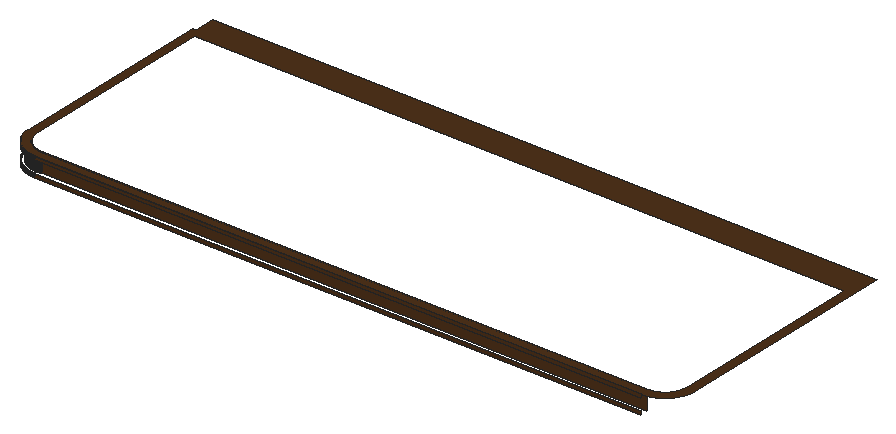
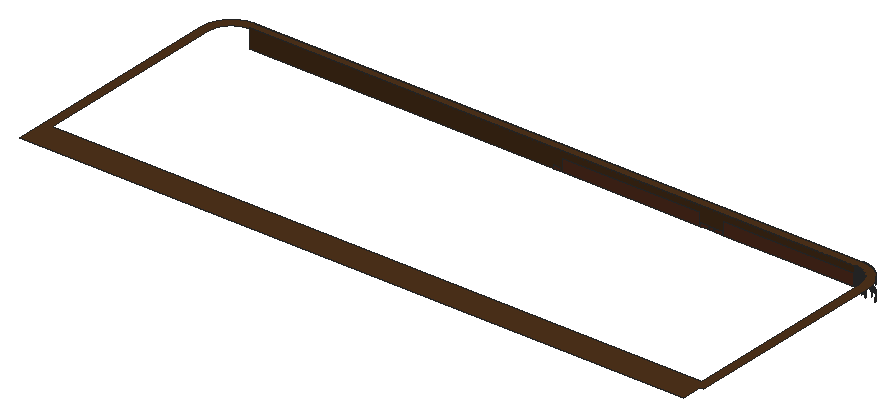
# SketchUp Ruby script. Lengths in inches.
U = 1.inch
M = Sketchup.active_model
def pt(a) = Geom::Point3d.new(a.map { |v| v * U })
def face(e, loops, mat)
  f = e.add_face(loops[0].map { |a| pt(a) })
  loops[1..].each { |l| e.add_face(l.map { |a| pt(a) }).erase! }
  f.material = f.back_material = mat if mat
  f
end
# faces: each face lists its corners as indices into pts; further lists are holes
def faces(e, pts, list, mat = nil) = list.each { |f| face(e, (f[0].is_a?(Array) ? f : [f]).map { |l| l.map { |i| pts[i] } }, mat) }
# xy, xz, yz: faces in a plane at the given z, y or x. An outline is a flat list of corners, or four numbers for a rectangle; further outlines are holes
def ring(l) = l.size == 4 ? [[l[0], l[1]], [l[2], l[1]], [l[2], l[3]], [l[0], l[3]]] : l.each_slice(2).to_a
def flat(e, list, mat, &to3) = list.each { |f| face(e, (f[0].is_a?(Array) ? f : [f]).map { |l| ring(l).map { |u, v| to3.(u, v) } }, mat) }
def xy(e, z, list, mat = nil) = flat(e, list, mat) { |x, y| [x, y, z] }
def xz(e, y, list, mat = nil) = flat(e, list, mat) { |x, z| [x, y, z] }
def yz(e, x, list, mat = nil) = flat(e, list, mat) { |y, z| [x, y, z] }
def lines(e, pts, list) = list.each { |a, b| e.add_line(pt(pts[a]), pt(pts[b])) }
# prism: a flat outline (further loops are holes) pulled along v
def prism(e, loops, v, mat = nil)
  f = face(e, loops, mat); d = Geom::Vector3d.new(v.map { |x| x * U })
  f.pushpull(f.normal.samedirection?(d) ? d.length : -d.length)
end
def box(e, o, s, mat = nil) = prism(e, [[o, [o[0] + s[0], o[1], o[2]], [o[0] + s[0], o[1] + s[1], o[2]], [o[0], o[1] + s[1], o[2]]]], [0, 0, s[2]], mat)
def at(x, y, z, deg = 0) = Geom::Transformation.translation(pt([x, y, z])) * Geom::Transformation.rotation(ORIGIN, Z_AXIS, deg.degrees)
def axes(o, x, y, z) = Geom::Transformation.new([*x, 0, *y, 0, *z, 0, *pt(o).to_a, 1])
def part(name) = M.definitions.add(name)
# library, detail: a bought-in or finely detailed component or shape, given as its bounding box
def library(name, o, s) = part(name).tap { |d| box(d.entities, o, s) }
def detail(e, o, s) = box(e.add_group.entities, o, s)
def put(e, d, t, mat = nil) = e.add_instance(d, t).tap { |i| i.material = mat if mat }
def group(e, t, mat = nil) = e.add_group.tap { |g| g.transformation = t; g.material = mat if mat }.entities
root = M.entities
M.materials.add("1799 AP 8574 BURNISHED CARAMEL").color = [140, 96, 69]
M.materials.add("1816 AP K197 Dark Kaapi-N").color = [79, 50, 27]
M.materials.add("[Wood Cherry Original]1").color = [93, 50, 33]
xy(root,401,[[[65.76,78,420.24,78,420.47,78.01,420.71,78.01,420.94,78.02,421.18,78.04,421.41,78.06,421.65,78.08,421.88,78.1,422.12,78.125,422.35,78.15,422.58,78.1875,422.82,78.22,423.28,78.3,423.51,78.35,423.74,78.39,423.97,78.44,424.2,78.5,424.43,78.55,424.66,78.61,424.89,78.68,425.11,78.74,425.34,78.81,425.5625,78.88,425.79,78.96,426.01,79.03,426.23,79.11,426.45,79.2,426.67,79.28,427.11,79.46,427.32,79.56,427.54,79.65,427.75,79.75,427.96,79.86,428.17,79.96,428.59,80.18,428.8,80.3,429,80.41,429.4,80.65,429.61,80.78,429.8,80.9,430,81.03,430.2,81.17,430.39,81.3,430.58,81.4375,430.77,81.58,430.96,81.72,431.14,81.86,431.33,82.01,431.51,82.16,431.69,82.3125,431.87,82.47,432.04,82.625,432.22,82.78,432.39,82.94,432.56,83.11,432.73,83.27,432.89,83.44,433.06,83.61,433.22,83.78,433.375,83.96,433.53,84.13,433.6875,84.31,433.84,84.49,433.99,84.67,434.14,84.86,434.28,85.04,434.42,85.23,434.5625,85.42,434.7,85.61,434.83,85.8,434.97,86,435.1,86.2,435.22,86.39,435.35,86.6,435.59,87,435.7,87.2,435.82,87.41,436.04,87.83,436.14,88.04,436.25,88.25,436.35,88.46,436.44,88.68,436.54,88.89,436.72,89.33,436.8,89.55,436.89,89.77,436.97,89.99,437.04,90.21,437.12,90.4375,437.19,90.66,437.26,90.89,437.32,91.11,437.39,91.34,437.45,91.57,437.5,91.8,437.56,92.03,437.61,92.26,437.65,92.49,437.7,92.72,437.78,93.18,437.8125,93.42,437.85,93.65,437.875,93.88,437.9,94.12,437.92,94.35,437.94,94.59,437.96,94.82,437.98,95.06,437.99,95.29,437.99,95.53,438,95.76,438,228,50,228,50,216,48,216,48,95.76,48.01,95.53,48.01,95.29,48.02,95.06,48.04,94.82,48.06,94.59,48.08,94.35,48.1,94.12,48.125,93.88,48.15,93.65,48.1875,93.42,48.22,93.18,48.3,92.72,48.35,92.49,48.39,92.26,48.44,92.03,48.5,91.8,48.55,91.57,48.61,91.34,48.68,91.11,48.74,90.89,48.81,90.66,48.88,90.4375,48.96,90.21,49.03,89.99,49.11,89.77,49.2,89.55,49.28,89.33,49.46,88.89,49.56,88.68,49.65,88.46,49.75,88.25,49.86,88.04,49.96,87.83,50.18,87.41,50.3,87.2,50.41,87,50.65,86.6,50.78,86.39,50.9,86.2,51.03,86,51.17,85.8,51.3,85.61,51.4375,85.42,51.58,85.23,51.72,85.04,51.86,84.86,52.01,84.67,52.16,84.49,52.3125,84.31,52.47,84.13,52.625,83.96,52.78,83.78,52.94,83.61,53.11,83.44,53.27,83.27,53.44,83.11,53.61,82.94,53.78,82.78,53.96,82.625,54.13,82.47,54.31,82.3125,54.49,82.16,54.67,82.01,54.86,81.86,55.04,81.72,55.23,81.58,55.42,81.4375,55.61,81.3,55.8,81.17,56,81.03,56.2,80.9,56.39,80.78,56.6,80.65,57,80.41,57.2,80.3,57.41,80.18,57.83,79.96,58.04,79.86,58.25,79.75,58.46,79.65,58.68,79.56,58.89,79.46,59.33,79.28,59.55,79.2,59.77,79.11,59.99,79.03,60.21,78.96,60.4375,78.88,60.66,78.81,60.89,78.74,61.11,78.68,61.34,78.61,61.57,78.55,61.8,78.5,62.03,78.44,62.26,78.39,62.49,78.35,62.72,78.3,63.18,78.22,63.42,78.1875,63.65,78.15,63.88,78.125,64.12,78.1,64.35,78.08,64.59,78.06,64.82,78.04,65.06,78.02,65.29,78.01,65.53,78.01],[65.66,83,64.81,83.05,64.13,83.13,63.97,83.16,63.8,83.1875,63.63,83.22,63.46,83.25,63.3,83.28,63.13,83.32,62.97,83.36,62.8,83.4,62.64,83.44,62.47,83.49,62.31,83.54,62.14,83.58,61.98,83.64,61.82,83.69,61.66,83.75,61.5,83.8,61.34,83.86,61.18,83.93,61.03,83.99,60.87,84.06,60.71,84.125,60.56,84.19,60.4,84.27,60.25,84.34,59.5,84.74,59.35,84.83,59.21,84.92,59.0625,85.01,58.92,85.1,58.78,85.19,58.64,85.29,58.5,85.38,58.22,85.58,58.09,85.6875,57.95,85.79,57.82,85.9,57.6875,86.01,57.56,86.11,57.43,86.23,57.3,86.34,57.18,86.45,57.05,86.57,56.93,86.6875,56.81,86.81,56.6875,86.93,56.57,87.05,56.45,87.18,56.34,87.3,56.23,87.43,56.11,87.56,56.01,87.6875,55.9,87.82,55.79,87.95,55.6875,88.09,55.58,88.22,55.38,88.5,55.29,88.64,55.19,88.78,55.1,88.92,55.01,89.0625,54.92,89.21,54.83,89.35,54.74,89.5,54.34,90.25,54.27,90.4,54.19,90.56,54.125,90.71,54.06,90.87,53.99,91.03,53.93,91.18,53.86,91.34,53.8,91.5,53.75,91.66,53.69,91.82,53.64,91.98,53.58,92.14,53.54,92.31,53.49,92.47,53.44,92.64,53.4,92.8,53.36,92.97,53.32,93.13,53.28,93.3,53.25,93.46,53.22,93.63,53.1875,93.8,53.16,93.97,53.13,94.13,53.05,94.81,53,95.66,53,211,433,211,433,95.66,432.95,94.81,432.87,94.13,432.84,93.97,432.8125,93.8,432.78,93.63,432.75,93.46,432.72,93.3,432.68,93.13,432.64,92.97,432.6,92.8,432.56,92.64,432.51,92.47,432.46,92.31,432.42,92.14,432.36,91.98,432.31,91.82,432.25,91.66,432.2,91.5,432.14,91.34,432.07,91.18,432.01,91.03,431.94,90.87,431.875,90.71,431.81,90.56,431.73,90.4,431.66,90.25,431.26,89.5,431.17,89.35,431.08,89.21,430.99,89.0625,430.9,88.92,430.81,88.78,430.71,88.64,430.62,88.5,430.42,88.22,430.3125,88.09,430.21,87.95,430.1,87.82,429.99,87.6875,429.89,87.56,429.77,87.43,429.66,87.3,429.55,87.18,429.43,87.05,429.3125,86.93,429.19,86.81,429.07,86.6875,428.95,86.57,428.82,86.45,428.7,86.34,428.57,86.23,428.44,86.11,428.3125,86.01,428.18,85.9,428.05,85.79,427.91,85.6875,427.78,85.58,427.5,85.38,427.36,85.29,427.22,85.19,427.08,85.1,426.9375,85.01,426.79,84.92,426.65,84.83,426.5,84.74,425.75,84.34,425.6,84.27,425.44,84.19,425.29,84.125,425.13,84.06,424.97,83.99,424.82,83.93,424.66,83.86,424.5,83.8,424.34,83.75,424.18,83.69,424.02,83.64,423.86,83.58,423.69,83.54,423.53,83.49,423.36,83.44,423.2,83.4,423.03,83.36,422.87,83.32,422.7,83.28,422.54,83.25,422.37,83.22,422.2,83.1875,422.03,83.16,421.87,83.13,421.19,83.05,420.34,83]]],"1816 AP K197 Dark Kaapi-N")
xz(root,78,[[65.76,390,66,392],[66,390,420,392],[65.76,399,66,401],[66,399,420,401]],"1816 AP K197 Dark Kaapi-N")
xz(root,78.01,[[65.29,390,65.53,392],[65.29,399,65.53,401]],"1816 AP K197 Dark Kaapi-N")
xz(root,80,[[65.79,392,66.01,399]],"1799 AP 8574 BURNISHED CARAMEL")
xz(root,80.01,[[65.37,392,65.58,399]],"1799 AP 8574 BURNISHED CARAMEL")
xz(root,83,[[65.66,390,65.83,401],[65.83,390,66.02,401],[66.02,390,419.98,401]],"1816 AP K197 Dark Kaapi-N")
xz(root,83,[[65.66,391,65.83,398],[65.83,391,66.02,398]],"[Wood Cherry Original]1")
xz(root,84.5,[[66.02,391,141.25,398],[142.75,391,146.75,392.75],[147.75,391,149.75,392.75],[150.75,391,154.75,392.75],[156.25,391,235.5,398],
  [237,391,241,392.75]],"[Wood Cherry Original]1")
p = [[64.59,78.06,390],[64.82,78.04,390],[64.82,78.04,392],[64.59,78.06,392],[65.06,78.02,390],[65.06,78.02,392],
  [65.29,78.01,390],[65.29,78.01,392],[65.53,78.01,390],[65.76,78,390],[65.76,78,392],[65.53,78.01,392],
  [63.65,78.15,390],[63.88,78.125,390],[63.88,78.125,392],[63.65,78.15,392],[64.12,78.1,390],[64.12,78.1,392],
  [64.35,78.08,390],[64.35,78.08,392],[62.95,78.26,390],[63.18,78.22,390],[63.18,78.22,392],[62.95,78.26,392],
  [63.42,78.1875,390],[63.42,78.1875,392],[62.26,78.39,390],[62.49,78.35,390],[62.49,78.35,392],[62.26,78.39,392],
  [62.72,78.3,390],[62.72,78.3,392],[61.8,78.5,390],[62.03,78.44,390],[62.03,78.44,392],[61.8,78.5,392],
  [61.57,78.55,390],[61.57,78.55,392],[61.11,78.68,390],[61.34,78.61,390],[61.34,78.61,392],[61.11,78.68,392],
  [60.66,78.81,390],[60.89,78.74,390],[60.89,78.74,392],[60.66,78.81,392],[60.4375,78.88,390],[60.4375,78.88,392],
  [60.21,78.96,390],[60.21,78.96,392],[59.77,79.11,390],[59.99,79.03,390],[59.99,79.03,392],[59.77,79.11,392],
  [59.55,79.2,390],[59.55,79.2,392],[59.33,79.28,390],[59.33,79.28,392],[59.11,79.37,390],[59.11,79.37,392],
  [58.89,79.46,390],[58.89,79.46,392],[58.68,79.56,390],[58.68,79.56,392],[58.46,79.65,390],[58.46,79.65,392],
  [58.25,79.75,390],[58.25,79.75,392],[58.04,79.86,390],[58.04,79.86,392],[57.83,79.96,390],[57.83,79.96,392],
  [57.62,80.07,390],[57.62,80.07,392],[57.41,80.18,390],[57.41,80.18,392],[57.2,80.3,390],[57.2,80.3,392],
  [57,80.41,390],[57,80.41,392],[56.8,80.53,390],[56.8,80.53,392],[56.6,80.65,390],[56.6,80.65,392],
  [56.39,80.78,390],[56.39,80.78,392],[56.2,80.9,390],[56.2,80.9,392],[56,81.03,390],[56,81.03,392],
  [55.8,81.17,390],[55.8,81.17,392],[55.61,81.3,390],[55.61,81.3,392],[55.42,81.4375,390],[55.42,81.4375,392],
  [55.23,81.58,390],[55.23,81.58,392],[55.04,81.72,390],[55.04,81.72,392],[54.86,81.86,390],[54.86,81.86,392],
  [54.67,82.01,390],[54.67,82.01,392],[54.49,82.16,390],[54.49,82.16,392],[54.31,82.3125,390],[54.31,82.3125,392],
  [54.13,82.47,390],[54.13,82.47,392],[53.96,82.625,390],[53.96,82.625,392],[53.78,82.78,390],[53.78,82.78,392],
  [53.61,82.94,390],[53.61,82.94,392],[53.44,83.11,390],[53.44,83.11,392],[64.81,83.05,401],[64.98,83.04,401],
  [64.98,83.04,390],[64.81,83.05,390],[65.15,83.03,401],[65.15,83.03,390],[65.32,83.02,401],[65.32,83.02,390],
  [65.49,83.01,401],[65.49,83.01,390],[65.66,83,401],[65.66,83,390],[53.27,83.27,390],[53.27,83.27,392],
  [63.97,83.16,401],[64.13,83.13,401],[64.13,83.13,390],[63.97,83.16,390],[64.3,83.11,401],[64.3,83.11,390],
  [64.47,83.09,401],[64.47,83.09,390],[64.64,83.07,401],[64.64,83.07,390],[63.3,83.28,401],[63.46,83.25,401],
  [63.46,83.25,390],[63.3,83.28,390],[63.63,83.22,401],[63.63,83.22,390],[63.8,83.1875,401],[63.8,83.1875,390],
  [53.11,83.44,390],[53.11,83.44,392],[62.97,83.36,401],[63.13,83.32,401],[63.13,83.32,390],[62.97,83.36,390],
  [52.94,83.61,390],[52.94,83.61,392],[62.47,83.49,401],[62.64,83.44,401],[62.64,83.44,390],[62.47,83.49,390],
  [62.8,83.4,401],[62.8,83.4,390],[62.14,83.58,401],[62.31,83.54,401],[62.31,83.54,390],[62.14,83.58,390],
  [52.78,83.78,390],[52.78,83.78,392],[61.82,83.69,401],[61.98,83.64,401],[61.98,83.64,390],[61.82,83.69,390],
  [61.5,83.8,401],[61.66,83.75,401],[61.66,83.75,390],[61.5,83.8,390],[52.625,83.96,390],[52.625,83.96,392],
  [61.34,83.86,401],[61.34,83.86,390],[61.03,83.99,401],[61.18,83.93,401],[61.18,83.93,390],[61.03,83.99,390],
  [52.47,84.13,390],[52.47,84.13,392],[60.87,84.06,401],[60.87,84.06,390],[52.3125,84.31,390],[52.3125,84.31,392],
  [60.56,84.19,401],[60.71,84.125,401],[60.71,84.125,390],[60.56,84.19,390],[60.4,84.27,401],[60.4,84.27,390],
  [52.16,84.49,390],[52.16,84.49,392],[60.1,84.42,401],[60.25,84.34,401],[60.25,84.34,390],[60.1,84.42,390],
  [59.95,84.5,401],[59.95,84.5,390],[52.01,84.67,390],[52.01,84.67,392],[59.8,84.58,401],[59.8,84.58,390],
  [59.65,84.66,401],[59.65,84.66,390],[51.86,84.86,390],[51.86,84.86,392],[59.35,84.83,401],[59.5,84.74,401],
  [59.5,84.74,390],[59.35,84.83,390],[59.21,84.92,401],[59.21,84.92,390],[51.72,85.04,390],[51.72,85.04,392],
  [59.0625,85.01,401],[59.0625,85.01,390],[51.58,85.23,390],[51.58,85.23,392],[58.92,85.1,401],[58.92,85.1,390],
  [58.78,85.19,401],[58.78,85.19,390],[51.4375,85.42,390],[51.4375,85.42,392],[58.64,85.29,401],[58.64,85.29,390],
  [58.5,85.38,401],[58.5,85.38,390],[51.3,85.61,390],[51.3,85.61,392],[58.36,85.48,401],[58.36,85.48,390],
  [58.22,85.58,401],[58.22,85.58,390],[51.17,85.8,390],[51.17,85.8,392],[58.09,85.6875,401],[58.09,85.6875,390],
  [57.95,85.79,401],[57.95,85.79,390],[51.03,86,390],[51.03,86,392],[57.82,85.9,401],[57.82,85.9,390],
  [57.6875,86.01,401],[57.6875,86.01,390],[50.9,86.2,390],[50.9,86.2,392],[57.56,86.11,401],[57.56,86.11,390],
  [57.43,86.23,401],[57.43,86.23,390],[50.78,86.39,390],[50.78,86.39,392],[57.3,86.34,401],[57.3,86.34,390],
  [57.18,86.45,401],[57.18,86.45,390],[50.65,86.6,390],[50.65,86.6,392],[57.05,86.57,401],[57.05,86.57,390],
  [50.53,86.8,390],[50.53,86.8,392],[56.93,86.6875,401],[56.93,86.6875,390],[56.81,86.81,401],[56.81,86.81,390],
  [50.41,87,390],[50.41,87,392],[56.6875,86.93,401],[56.6875,86.93,390],[56.57,87.05,401],[56.57,87.05,390],
  [50.3,87.2,390],[50.3,87.2,392],[56.45,87.18,401],[56.45,87.18,390],[50.18,87.41,390],[50.18,87.41,392],
  [56.34,87.3,401],[56.34,87.3,390],[56.23,87.43,401],[56.23,87.43,390],[50.07,87.62,390],[50.07,87.62,392],
  [56.11,87.56,401],[56.11,87.56,390],[49.96,87.83,390],[49.96,87.83,392],[56.01,87.6875,401],[56.01,87.6875,390],
  [55.9,87.82,401],[55.9,87.82,390],[49.86,88.04,390],[49.86,88.04,392],[55.79,87.95,401],[55.79,87.95,390],
  [49.75,88.25,390],[49.75,88.25,392],[55.6875,88.09,401],[55.6875,88.09,390],[64.81,83.05,391],[64.98,83.04,391],
  [64.98,83.04,398],[64.81,83.05,398],[65.15,83.03,391],[65.15,83.03,398],[65.32,83.02,391],[65.32,83.02,398],
  [65.49,83.01,391],[65.49,83.01,398],[65.66,83,391],[65.66,83,398],[63.97,83.16,391],[64.13,83.13,391],
  [64.13,83.13,398],[63.97,83.16,398],[64.3,83.11,391],[64.3,83.11,398],[64.47,83.09,391],[64.47,83.09,398],
  [64.64,83.07,391],[64.64,83.07,398],[63.3,83.28,391],[63.46,83.25,391],[63.46,83.25,398],[63.3,83.28,398],
  [63.63,83.22,391],[63.63,83.22,398],[63.8,83.1875,391],[63.8,83.1875,398],[62.97,83.36,391],[63.13,83.32,391],
  [63.13,83.32,398],[62.97,83.36,398],[62.47,83.49,391],[62.64,83.44,391],[62.64,83.44,398],[62.47,83.49,398],
  [62.8,83.4,391],[62.8,83.4,398],[62.14,83.58,391],[62.31,83.54,391],[62.31,83.54,398],[62.14,83.58,398],
  [61.82,83.69,391],[61.98,83.64,391],[61.98,83.64,398],[61.82,83.69,398],[61.5,83.8,391],[61.66,83.75,391],
  [61.66,83.75,398],[61.5,83.8,398],[61.34,83.86,391],[61.34,83.86,398],[61.03,83.99,391],[61.18,83.93,391],
  [61.18,83.93,398],[61.03,83.99,398],[60.87,84.06,391],[60.87,84.06,398],[60.56,84.19,391],[60.71,84.125,391],
  [60.71,84.125,398],[60.56,84.19,398],[60.4,84.27,391],[60.4,84.27,398],[60.1,84.42,391],[60.25,84.34,391],
  [60.25,84.34,398],[60.1,84.42,398],[59.95,84.5,391],[59.95,84.5,398],[59.8,84.58,391],[59.8,84.58,398],
  [59.65,84.66,391],[59.65,84.66,398],[64.3,84.64,392.75],[64,84.68,391],[63.74,84.74,392.75],[64.52,84.61,391],
  [64.52,84.61,392.75],[59.35,84.83,391],[59.5,84.74,391],[59.5,84.74,398],[59.35,84.83,398],[59.52,84.73,391],
  [63.48,84.78,391],[63.18,84.87,392.75],[59.21,84.92,391],[59.21,84.92,398],[62.97,84.91,391],[59.0625,85.01,391],
  [59.0625,85.01,398],[62.46,85.0625,391],[62.625,85.02,392.75],[58.92,85.1,391],[58.92,85.1,398],[62.08,85.2,392.75],
  [58.78,85.19,391],[58.78,85.19,398],[61.96,85.24,391],[58.64,85.29,391],[58.64,85.29,398],[61.47,85.43,391],
  [61.54,85.41,392.75],[58.5,85.38,391],[58.5,85.38,398],[58.36,85.48,391],[58.36,85.48,398],[60.99,85.66,391],
  [61.02,85.65,392.75],[58.22,85.58,391],[58.22,85.58,398],[58.09,85.6875,391],[58.09,85.6875,398],[60.52,85.9,392.75],
  [57.95,85.79,391],[57.95,85.79,398],[60.52,85.9,391],[57.82,85.9,391],[57.82,85.9,398],[57.6875,86.01,391],
  [57.6875,86.01,398],[57.56,86.11,391],[57.56,86.11,398],[57.43,86.23,391],[57.52,86.15,391],[57.43,86.23,398],
  [57.3,86.34,391],[57.3,86.34,398],[57.18,86.45,391],[57.18,86.45,398],[57.05,86.57,391],[57.05,86.57,398],
  [59.49,86.52,391],[59.24,86.7,391],[59.24,86.7,392.75],[59.49,86.52,392.75],[59.52,86.5,391],[59.52,86.5,392.75],
  [56.93,86.6875,391],[56.93,86.6875,398],[56.81,86.81,391],[56.81,86.81,398],[59.12,86.79,391],[59.12,86.79,392.75],
  [56.6875,86.93,391],[56.6875,86.93,398],[58.88,86.97,391],[58.88,86.97,392.75],[56.57,87.05,391],[56.57,87.05,398],
  [58.65,87.16,391],[58.65,87.16,392.75],[56.45,87.18,391],[56.45,87.18,398],[56.34,87.3,391],[56.34,87.3,398],
  [58.42,87.35,391],[58.42,87.35,392.75],[56.23,87.43,391],[56.23,87.43,398],[56.11,87.56,391],[56.11,87.56,398],
  [58.19,87.56,391],[58.19,87.56,392.75],[56.01,87.6875,391],[56.01,87.6875,398],[58.08,87.66,391],[58.08,87.66,392.75],
  [55.9,87.82,391],[55.9,87.82,398],[57.87,87.87,391],[57.87,87.87,392.75],[55.79,87.95,391],[55.79,87.95,398],
  [57.66,88.08,391],[57.66,88.08,392.75],[55.6875,88.09,391],[55.6875,88.09,398],[64.54,80.07,392],[64.74,80.05,392],
  [64.74,80.05,399],[64.54,80.07,399],[64.95,80.03,392],[64.95,80.03,399],[65.16,80.02,392],[65.16,80.02,399],
  [65.37,80.01,392],[65.37,80.01,399],[65.58,80.01,392],[65.79,80,392],[65.79,80,399],[65.58,80.01,399],
  [63.7,80.17,392],[63.91,80.14,392],[63.91,80.14,399],[63.7,80.17,399],[64.12,80.11,392],[64.12,80.11,399],
  [64.33,80.09,392],[64.33,80.09,399],[63.08,80.27,392],[63.29,80.23,392],[63.29,80.23,399],[63.08,80.27,399],
  [63.5,80.2,392],[63.5,80.2,399],[62.47,80.39,392],[62.67,80.35,392],[62.67,80.35,399],[62.47,80.39,399],
  [62.88,80.31,392],[62.88,80.31,399],[62.0625,80.49,392],[62.26,80.44,392],[62.26,80.44,399],[62.0625,80.49,399],
  [61.66,80.6,392],[61.86,80.55,392],[61.86,80.55,399],[61.66,80.6,399],[61.46,80.66,392],[61.46,80.66,399],
  [61.06,80.78,392],[61.26,80.72,392],[61.26,80.72,399],[61.06,80.78,399],[60.66,80.92,392],[60.86,80.85,392],
  [60.86,80.85,399],[60.66,80.92,399],[60.46,80.99,392],[60.46,80.99,399],[60.27,81.0625,392],[60.27,81.0625,399],
  [59.88,81.22,392],[60.07,81.14,392],[60.07,81.14,399],[59.88,81.22,399],[59.68,81.3,392],[59.68,81.3,399],
  [59.49,81.38,392],[59.49,81.38,399],[59.3,81.47,392],[59.3,81.47,399],[59.11,81.56,392],[59.11,81.56,399],
  [58.92,81.65,392],[58.92,81.65,399],[58.55,81.84,392],[58.74,81.74,392],[58.74,81.74,399],[58.55,81.84,399],
  [58.37,81.9375,392],[58.37,81.9375,399],[58.18,82.04,392],[58.18,82.04,399],[58,82.14,392],[58,82.14,399],
  [57.82,82.25,392],[57.82,82.25,399],[57.64,82.36,392],[57.64,82.36,399],[57.46,82.47,392],[57.46,82.47,399],
  [57.29,82.58,392],[57.29,82.58,399],[57.11,82.7,392],[57.11,82.7,399],[56.9375,82.8125,392],[56.9375,82.8125,399],
  [56.77,82.93,392],[56.77,82.93,399],[56.6,83.06,392],[56.6,83.06,399],[56.43,83.18,392],[56.43,83.18,399],
  [56.26,83.31,392],[56.26,83.31,399],[56.09,83.43,392],[56.09,83.43,399],[55.93,83.57,392],[55.93,83.57,399],
  [55.77,83.7,392],[55.77,83.7,399],[55.61,83.83,392],[55.61,83.83,399],[55.45,83.97,392],[55.45,83.97,399],
  [55.29,84.11,392],[55.29,84.11,399],[55.14,84.25,392],[55.14,84.25,399],[54.99,84.39,392],[54.99,84.39,399],
  [54.84,84.54,392],[54.84,84.54,399],[54.6875,84.6875,392],[54.6875,84.6875,399],[54.54,84.84,392],[54.54,84.84,399],
  [54.39,84.99,392],[54.39,84.99,399],[54.25,85.14,392],[54.25,85.14,399],[54.11,85.29,392],[54.11,85.29,399],
  [53.97,85.45,392],[53.97,85.45,399],[53.83,85.61,392],[53.83,85.61,399],[53.7,85.77,392],[53.7,85.77,399],
  [53.57,85.93,392],[53.57,85.93,399],[53.43,86.09,392],[53.43,86.09,399],[53.31,86.26,392],[53.31,86.26,399],
  [53.18,86.43,392],[53.18,86.43,399],[53.06,86.6,392],[53.06,86.6,399],[52.93,86.77,392],[52.93,86.77,399],
  [52.8125,86.9375,392],[52.8125,86.9375,399],[52.7,87.11,392],[52.7,87.11,399],[52.58,87.29,392],[52.58,87.29,399],
  [52.47,87.46,392],[52.47,87.46,399],[52.36,87.64,392],[52.36,87.64,399],[52.25,87.82,392],[52.25,87.82,399],
  [52.14,88,392],[52.14,88,399],[52.04,88.18,392],[52.04,88.18,399],[64.59,78.06,399],[64.82,78.04,399],
  [64.82,78.04,401],[64.59,78.06,401],[65.06,78.02,399],[65.06,78.02,401],[65.29,78.01,399],[65.29,78.01,401],
  [65.53,78.01,399],[65.76,78,399],[65.76,78,401],[65.53,78.01,401],[63.65,78.15,399],[63.88,78.125,399],
  [63.88,78.125,401],[63.65,78.15,401],[64.12,78.1,399],[64.12,78.1,401],[64.35,78.08,399],[64.35,78.08,401],
  [62.95,78.26,399],[63.18,78.22,399],[63.18,78.22,401],[62.95,78.26,401],[63.42,78.1875,399],[63.42,78.1875,401],
  [62.26,78.39,399],[62.49,78.35,399],[62.49,78.35,401],[62.26,78.39,401],[62.72,78.3,399],[62.72,78.3,401],
  [61.8,78.5,399],[62.03,78.44,399],[62.03,78.44,401],[61.8,78.5,401],[61.57,78.55,399],[61.57,78.55,401],
  [61.11,78.68,399],[61.34,78.61,399],[61.34,78.61,401],[61.11,78.68,401],[60.66,78.81,399],[60.89,78.74,399],
  [60.89,78.74,401],[60.66,78.81,401],[60.4375,78.88,399],[60.4375,78.88,401],[60.21,78.96,399],[60.21,78.96,401],
  [59.77,79.11,399],[59.99,79.03,399],[59.99,79.03,401],[59.77,79.11,401],[59.55,79.2,399],[59.55,79.2,401],
  [59.33,79.28,399],[59.33,79.28,401],[59.11,79.37,399],[59.11,79.37,401],[58.89,79.46,399],[58.89,79.46,401],
  [58.68,79.56,399],[58.68,79.56,401],[58.46,79.65,399],[58.46,79.65,401],[58.25,79.75,399],[58.25,79.75,401],
  [58.04,79.86,399],[58.04,79.86,401],[57.83,79.96,399],[57.83,79.96,401],[57.62,80.07,399],[57.62,80.07,401],
  [57.41,80.18,399],[57.41,80.18,401],[57.2,80.3,399],[57.2,80.3,401],[57,80.41,399],[57,80.41,401],
  [56.8,80.53,399],[56.8,80.53,401],[56.6,80.65,399],[56.6,80.65,401],[56.39,80.78,399],[56.39,80.78,401],
  [56.2,80.9,399],[56.2,80.9,401],[56,81.03,399],[56,81.03,401],[55.8,81.17,399],[55.8,81.17,401],
  [55.61,81.3,399],[55.61,81.3,401],[55.42,81.4375,399],[55.42,81.4375,401],[55.23,81.58,399],[55.23,81.58,401],
  [55.04,81.72,399],[55.04,81.72,401],[54.86,81.86,399],[54.86,81.86,401],[54.67,82.01,399],[54.67,82.01,401],
  [54.49,82.16,399],[54.49,82.16,401],[54.31,82.3125,399],[54.31,82.3125,401],[54.13,82.47,399],[54.13,82.47,401],
  [53.96,82.625,399],[53.96,82.625,401],[53.78,82.78,399],[53.78,82.78,401],[53.61,82.94,399],[53.61,82.94,401],
  [53.44,83.11,399],[53.44,83.11,401],[53.27,83.27,399],[53.27,83.27,401],[53.11,83.44,399],[53.11,83.44,401],
  [52.94,83.61,399],[52.94,83.61,401],[52.78,83.78,399],[52.78,83.78,401],[52.625,83.96,399],[52.625,83.96,401],
  [52.47,84.13,399],[52.47,84.13,401],[52.3125,84.31,399],[52.3125,84.31,401],[52.16,84.49,399],[52.16,84.49,401],
  [52.01,84.67,399],[52.01,84.67,401],[51.86,84.86,399],[51.86,84.86,401],[51.72,85.04,399],[51.72,85.04,401],
  [51.58,85.23,399],[51.58,85.23,401],[51.4375,85.42,399],[51.4375,85.42,401],[51.3,85.61,399],[51.3,85.61,401],
  [51.17,85.8,399],[51.17,85.8,401],[51.03,86,399],[51.03,86,401],[50.9,86.2,399],[50.9,86.2,401],
  [50.78,86.39,399],[50.78,86.39,401],[50.65,86.6,399],[50.65,86.6,401],[50.53,86.8,399],[50.53,86.8,401],
  [50.41,87,399],[50.41,87,401],[50.3,87.2,399],[50.3,87.2,401],[50.18,87.41,399],[50.18,87.41,401],
  [50.07,87.62,399],[50.07,87.62,401],[49.96,87.83,399],[49.96,87.83,401],[49.86,88.04,399],[49.86,88.04,401],
  [59.52,84.5,391],[57.52,84.5,391],[64.8,84.5625,391],[64.8,84.5625,392.75],[65.1,84.54,391],[65.1,84.54,392.75],
  [65.55,84.51,391],[65.55,84.51,392.75],[65.85,84.5,391],[65.85,84.5,392.75]]
faces(root,p,[[0,1,2,3],[1,4,5,2],[4,6,7,5],[8,9,10,11],[12,13,14,15],[13,16,17,14],[16,18,19,17],[18,0,3,19],
  [20,21,22,23],[21,24,25,22],[24,12,15,25],[26,27,28,29],[27,30,31,28],[30,20,23,31],[32,33,34,35],[33,26,29,34],
  [36,32,35,37],[38,39,40,41],[39,36,37,40],[42,43,44,45],[43,38,41,44],[46,42,45,47],[48,46,47,49],[50,51,52,53],
  [51,48,49,52],[54,50,53,55],[56,54,55,57],[58,56,57,59],[60,58,59,61],[62,60,61,63],[64,62,63,65],[66,64,65,67],
  [68,66,67,69],[70,68,69,71],[72,70,71,73],[74,72,73,75],[76,74,75,77],[78,76,77,79],[80,78,79,81],[82,80,81,83],
  [84,82,83,85],[86,84,85,87],[88,86,87,89],[90,88,89,91],[92,90,91,93],[94,92,93,95],[96,94,95,97],[98,96,97,99],
  [100,98,99,101],[102,100,101,103],[104,102,103,105],[106,104,105,107],[108,106,107,109],[110,108,109,111],[112,110,111,113],[114,112,113,115],
  [116,114,115,117],[118,119,120,121],[119,122,123,120],[122,124,125,123],[124,126,127,125],[126,128,129,127],[130,116,117,131],[132,133,134,135],
  [133,136,137,134],[136,138,139,137],[138,140,141,139],[140,118,121,141],[142,143,144,145],[143,146,147,144],[146,148,149,147],[148,132,135,149],
  [150,130,131,151],[152,153,154,155],[153,142,145,154],[156,150,151,157],[158,159,160,161],[159,162,163,160],[162,152,155,163],[164,165,166,167],
  [165,158,161,166],[168,156,157,169],[170,171,172,173],[171,164,167,172],[174,175,176,177],[175,170,173,176],[178,168,169,179],[180,174,177,181],
  [182,183,184,185],[183,180,181,184],[186,178,179,187],[188,182,185,189],[190,186,187,191],[192,193,194,195],[193,188,189,194],[196,192,195,197],
  [198,190,191,199],[200,201,202,203],[201,196,197,202],[204,200,203,205],[206,198,199,207],[208,204,205,209],[210,208,209,211],[212,206,207,213],
  [214,215,216,217],[215,210,211,216],[218,214,217,219],[220,212,213,221],[222,218,219,223],[224,220,221,225],[226,222,223,227],[228,226,227,229],
  [230,224,225,231],[232,228,229,233],[234,232,233,235],[236,230,231,237],[238,234,235,239],[240,238,239,241],[242,236,237,243],[244,240,241,245],
  [246,244,245,247],[248,242,243,249],[250,246,247,251],[252,250,251,253],[254,248,249,255],[256,252,253,257],[258,256,257,259],[260,254,255,261],
  [262,258,259,263],[264,262,263,265],[266,260,261,267],[268,264,265,269],[270,266,267,271],[272,268,269,273],[274,272,273,275],[276,270,271,277],
  [278,274,275,279],[280,278,279,281],[282,276,277,283],[284,280,281,285],[286,282,283,287],[288,284,285,289],[290,288,289,291],[292,286,287,293],
  [294,290,291,295],[296,292,293,297],[298,294,295,299],[300,298,299,301],[302,296,297,303],[304,300,301,305],[306,302,303,307],[308,304,305,309],
  [652,653,654,655],[653,656,657,654],[656,658,659,657],[660,661,662,663],[664,665,666,667],[665,668,669,666],[668,670,671,669],[670,652,655,671],
  [672,673,674,675],[673,676,677,674],[676,664,667,677],[678,679,680,681],[679,682,683,680],[682,672,675,683],[684,685,686,687],[685,678,681,686],
  [688,684,687,689],[690,691,692,693],[691,688,689,692],[694,695,696,697],[695,690,693,696],[698,694,697,699],[700,698,699,701],[702,703,704,705],
  [703,700,701,704],[706,702,705,707],[708,706,707,709],[710,708,709,711],[712,710,711,713],[714,712,713,715],[716,714,715,717],[718,716,717,719],
  [720,718,719,721],[722,720,721,723],[724,722,723,725],[726,724,725,727],[728,726,727,729],[730,728,729,731],[732,730,731,733],[734,732,733,735],
  [736,734,735,737],[738,736,737,739],[740,738,739,741],[742,740,741,743],[744,742,743,745],[746,744,745,747],[748,746,747,749],[750,748,749,751],
  [752,750,751,753],[754,752,753,755],[756,754,755,757],[758,756,757,759],[760,758,759,761],[762,760,761,763],[764,762,763,765],[766,764,765,767],
  [768,766,767,769],[770,768,769,771],[772,770,771,773],[774,772,773,775],[776,774,775,777],[778,776,777,779],[780,778,779,781],[782,780,781,783],
  [784,782,783,785],[786,784,785,787],[788,786,787,789],[790,788,789,791],[792,790,791,793],[794,792,793,795],[796,794,795,797],[798,796,797,799],
  [800,798,799,801],[802,800,801,803],[804,802,803,805],[806,804,805,807],[808,806,807,809],[810,808,809,811],[812,810,811,813],[814,812,813,815],
  [816,814,815,817],[818,816,817,819],[820,818,819,821]],"1816 AP K197 Dark Kaapi-N")
faces(root,p,[[310,311,312,313],[311,314,315,312],[314,316,317,315],[316,318,319,317],[318,320,321,319],[322,323,324,325],[323,326,327,324],[326,328,329,327],
  [328,330,331,329],[330,310,313,331],[332,333,334,335],[333,336,337,334],[336,338,339,337],[338,322,325,339],[340,341,342,343],[341,332,335,342],
  [344,345,346,347],[345,348,349,346],[348,340,343,349],[350,351,352,353],[351,344,347,352],[354,355,356,357],[355,350,353,356],[358,359,360,361],
  [359,354,357,360],[362,358,361,363],[364,365,366,367],[365,362,363,366],[368,364,367,369],[370,371,372,373],[371,368,369,372],[374,370,373,375],
  [376,377,378,379],[377,374,375,378],[380,376,379,381],[382,380,381,383],[384,382,383,385],[386,387,388],[387,386,389],[390,389,386],
  [391,392,393,394],[392,395,384,385,393],[388,396,397],[396,388,387],[398,391,394,399],[400,397,396],[401,398,399,402],[403,404,400],
  [397,400,404],[405,401,402,406],[404,403,407],[408,405,406,409],[410,407,403],[411,408,409,412],[413,414,410],[407,410,414],
  [415,411,412,416],[417,415,416,418],[419,420,413],[414,413,420],[421,417,418,422],[423,421,422,424],[420,419,425],[426,423,424,427],
  [428,425,419],[429,426,427,430],[431,429,430,432],[433,431,432,434],[435,436,433,434,437],[438,435,437,439],[440,438,439,441],[442,440,441,443],
  [444,445,446,447],[448,444,447,449],[450,442,443,451],[452,450,451,453],[445,454,455,446],[456,452,453,457],[454,458,459,455],[460,456,457,461],
  [458,462,463,459],[464,460,461,465],[466,464,465,467],[462,468,469,463],[470,466,467,471],[472,470,471,473],[468,474,475,469],[476,472,473,477],
  [474,478,479,475],[480,476,477,481],[478,482,483,479],[484,480,481,485],[482,486,487,483],[488,484,485,489]],"[Wood Cherry Original]1")
faces(root,p,[[490,491,492,493],[491,494,495,492],[494,496,497,495],[496,498,499,497],[500,501,502,503],[504,505,506,507],[505,508,509,506],[508,510,511,509],
  [510,490,493,511],[512,513,514,515],[513,516,517,514],[516,504,507,517],[518,519,520,521],[519,522,523,520],[522,512,515,523],[524,525,526,527],
  [525,518,521,526],[528,529,530,531],[529,524,527,530],[532,528,531,533],[534,535,536,537],[535,532,533,536],[538,539,540,541],[539,534,537,540],
  [542,538,541,543],[544,542,543,545],[546,547,548,549],[547,544,545,548],[550,546,549,551],[552,550,551,553],[554,552,553,555],[556,554,555,557],
  [558,556,557,559],[560,561,562,563],[561,558,559,562],[564,560,563,565],[566,564,565,567],[568,566,567,569],[570,568,569,571],[572,570,571,573],
  [574,572,573,575],[576,574,575,577],[578,576,577,579],[580,578,579,581],[582,580,581,583],[584,582,583,585],[586,584,585,587],[588,586,587,589],
  [590,588,589,591],[592,590,591,593],[594,592,593,595],[596,594,595,597],[598,596,597,599],[600,598,599,601],[602,600,601,603],[604,602,603,605],
  [606,604,605,607],[608,606,607,609],[610,608,609,611],[612,610,611,613],[614,612,613,615],[616,614,615,617],[618,616,617,619],[620,618,619,621],
  [622,620,621,623],[624,622,623,625],[626,624,625,627],[628,626,627,629],[630,628,629,631],[632,630,631,633],[634,632,633,635],[636,634,635,637],
  [638,636,637,639],[640,638,639,641],[642,640,641,643],[644,642,643,645],[646,644,645,647],[648,646,647,649],[650,648,649,651]],"1799 AP 8574 BURNISHED CARAMEL")
lines(root,p,[[395,822],[436,823],[824,825],[826,827],[828,829],[830,831]])
